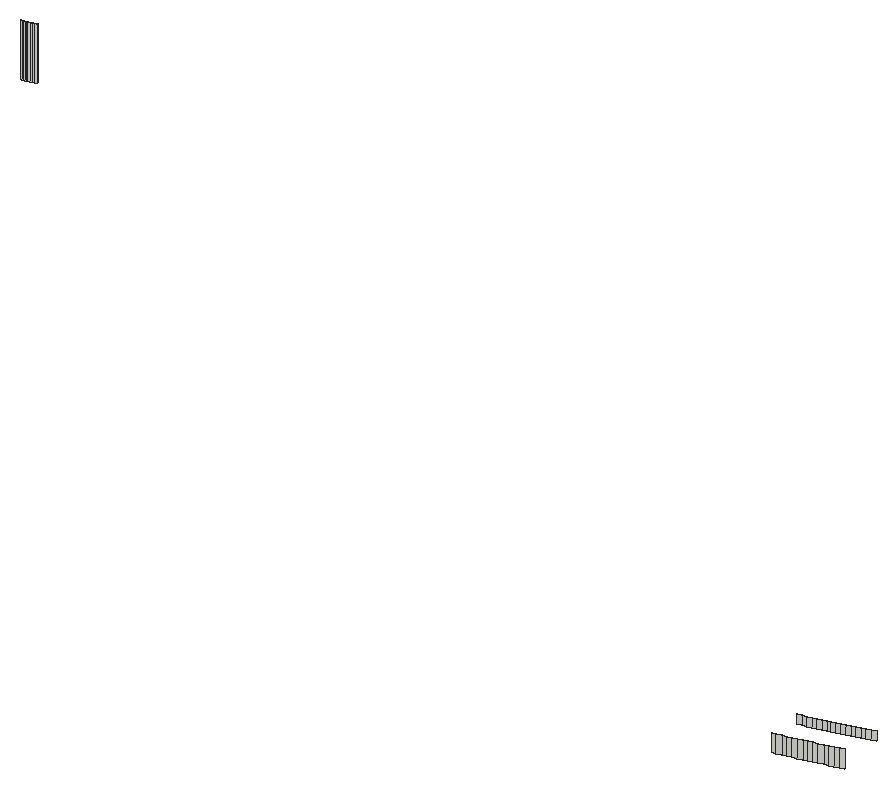
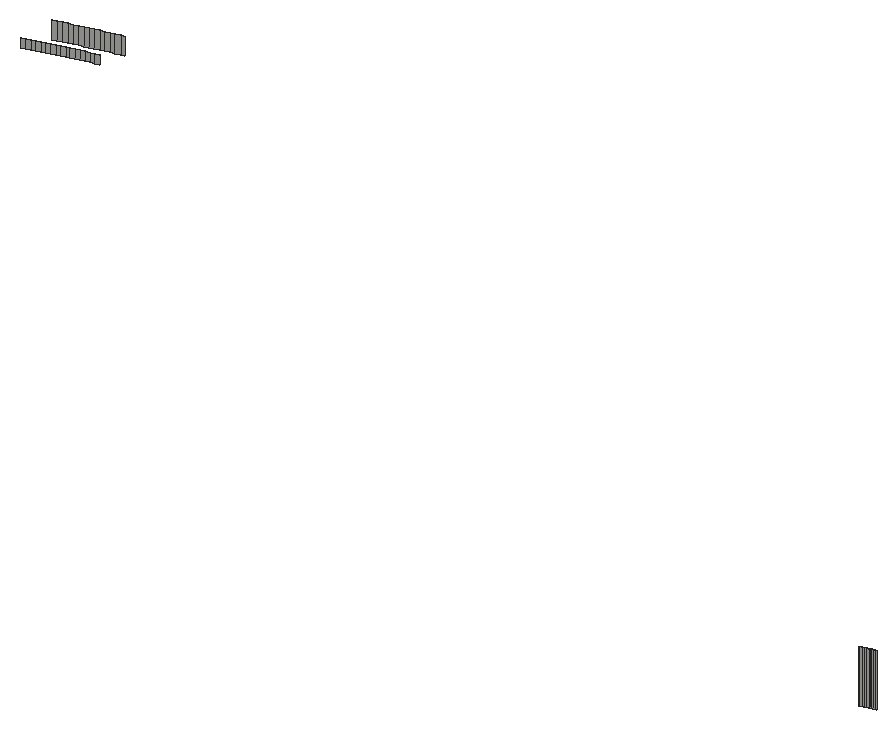
# SketchUp Ruby script. Lengths in inches.
U = 1.inch
M = Sketchup.active_model
def pt(a) = Geom::Point3d.new(a.map { |v| v * U })
def face(e, loops, mat)
  f = e.add_face(loops[0].map { |a| pt(a) })
  loops[1..].each { |l| e.add_face(l.map { |a| pt(a) }).erase! }
  f.material = f.back_material = mat if mat
  f
end
# faces: each face lists its corners as indices into pts; further lists are holes
def faces(e, pts, list, mat = nil) = list.each { |f| face(e, (f[0].is_a?(Array) ? f : [f]).map { |l| l.map { |i| pts[i] } }, mat) }
# xy, xz, yz: faces in a plane at the given z, y or x. An outline is a flat list of corners, or four numbers for a rectangle; further outlines are holes
def ring(l) = l.size == 4 ? [[l[0], l[1]], [l[2], l[1]], [l[2], l[3]], [l[0], l[3]]] : l.each_slice(2).to_a
def flat(e, list, mat, &to3) = list.each { |f| face(e, (f[0].is_a?(Array) ? f : [f]).map { |l| ring(l).map { |u, v| to3.(u, v) } }, mat) }
def xy(e, z, list, mat = nil) = flat(e, list, mat) { |x, y| [x, y, z] }
def xz(e, y, list, mat = nil) = flat(e, list, mat) { |x, z| [x, y, z] }
def yz(e, x, list, mat = nil) = flat(e, list, mat) { |y, z| [x, y, z] }
def lines(e, pts, list) = list.each { |a, b| e.add_line(pt(pts[a]), pt(pts[b])) }
# prism: a flat outline (further loops are holes) pulled along v
def prism(e, loops, v, mat = nil)
  f = face(e, loops, mat); d = Geom::Vector3d.new(v.map { |x| x * U })
  f.pushpull(f.normal.samedirection?(d) ? d.length : -d.length)
end
def box(e, o, s, mat = nil) = prism(e, [[o, [o[0] + s[0], o[1], o[2]], [o[0] + s[0], o[1] + s[1], o[2]], [o[0], o[1] + s[1], o[2]]]], [0, 0, s[2]], mat)
def at(x, y, z, deg = 0) = Geom::Transformation.translation(pt([x, y, z])) * Geom::Transformation.rotation(ORIGIN, Z_AXIS, deg.degrees)
def axes(o, x, y, z) = Geom::Transformation.new([*x, 0, *y, 0, *z, 0, *pt(o).to_a, 1])
def part(name) = M.definitions.add(name)
# library, detail: a bought-in or finely detailed component or shape, given as its bounding box
def library(name, o, s) = part(name).tap { |d| box(d.entities, o, s) }
def detail(e, o, s) = box(e.add_group.entities, o, s)
def put(e, d, t, mat = nil) = e.add_instance(d, t).tap { |i| i.material = mat if mat }
def group(e, t, mat = nil) = e.add_group.tap { |g| g.transformation = t; g.material = mat if mat }.entities
root = M.entities
xz(root,161,[[323.19,108,323.21,108.5]])
p = [[323.59,159.04,107.5],[323.38,159,107.5],[323.38,159,108.5],[323.59,159.04,108.5],[323.84,159.09,107.5],[323.84,159.09,108.5],
  [324.1,159.14,107.5],[324.1,159.14,108.5],[324.35,159.2,107.5],[324.35,159.2,108.5],[324.6,159.26,107.5],[324.6,159.26,108.5],
  [324.85,159.32,107.5],[324.85,159.32,108.5],[325.1,159.38,107.5],[325.1,159.38,108.5],[325.34,159.44,107.5],[325.34,159.44,108.5],
  [325.59,159.51,107.5],[325.59,159.51,108.5],[325.84,159.58,107.5],[325.84,159.58,108.5],[326.09,159.65,107.5],[326.09,159.65,108.5],
  [326.33,159.72,107.5],[326.33,159.72,108.5],[326.58,159.79,107.5],[326.58,159.79,108.5],[326.83,159.87,107.5],[326.83,159.87,108.5],
  [323.21,161,108],[323.44,161.05,108],[323.44,161.05,108.5],[323.21,161,108.5],[323.68,161.1,108],[323.68,161.1,108.5],
  [323.91,161.15,108],[323.91,161.15,108.5],[324.14,161.2,108],[324.14,161.2,108.5],[324.375,161.26,108],[324.375,161.26,108.5],
  [324.61,161.32,108],[324.61,161.32,108.5],[324.84,161.375,108],[324.84,161.375,108.5],[325.07,161.4375,108],[325.07,161.4375,108.5],
  [325.3,161.5,108],[325.3,161.5,108.5],[325.53,161.57,108],[325.53,161.57,108.5],[325.76,161.64,108],[325.76,161.64,108.5],
  [325.99,161.7,108],[325.99,161.7,108.5],[326.22,161.78,108],[326.22,161.78,108.5],[326.44,161.85,108],[326.44,161.85,108.5],
  [326.67,161.93,108],[326.67,161.93,108.5],[326.9,162,108],[326.9,162,108.5],[259.97,185.04,108],[259.89,185.03,108],
  [259.89,185.03,111],[259.97,185.04,111],[260.05,185.05,108],[260.05,185.05,111],[260.125,185.07,108],[260.125,185.07,111],
  [260.2,185.08,108],[260.2,185.08,111],[260.28,185.1,108],[260.28,185.1,111],[260.35,185.125,108],[260.35,185.125,111],
  [260.43,185.15,108],[260.43,185.15,111],[260.5,185.17,108],[260.5,185.17,111],[260.58,185.2,108],[260.58,185.2,111],
  [260.65,185.23,108],[260.65,185.23,111],[260.72,185.26,108],[260.72,185.26,111]]
faces(root,p,[[0,1,2,3],[4,0,3,5],[6,4,5,7],[8,6,7,9],[10,8,9,11],[12,10,11,13],[14,12,13,15],[16,14,15,17],
  [18,16,17,19],[20,18,19,21],[22,20,21,23],[24,22,23,25],[26,24,25,27],[28,26,27,29],[30,31,32,33],[31,34,35,32],
  [34,36,37,35],[36,38,39,37],[38,40,41,39],[40,42,43,41],[42,44,45,43],[44,46,47,45],[46,48,49,47],[48,50,51,49],
  [50,52,53,51],[52,54,55,53],[54,56,57,55],[56,58,59,57],[58,60,61,59],[60,62,63,61],[64,65,66,67],[68,64,67,69],
  [70,68,69,71],[72,70,71,73],[74,72,73,75],[76,74,75,77],[78,76,77,79],[80,78,79,81],[82,80,81,83],[84,82,83,85],
  [86,84,85,87]])
